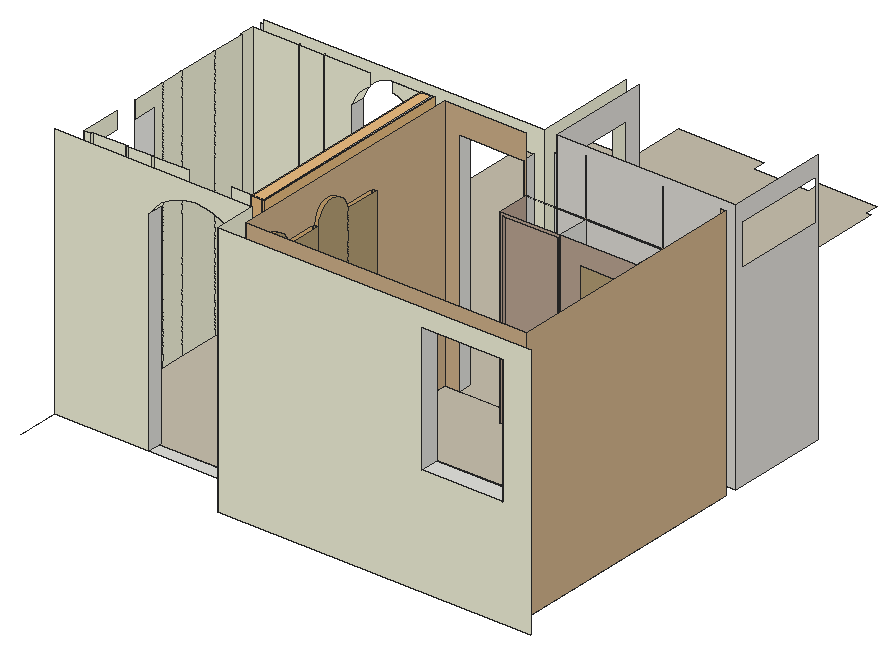
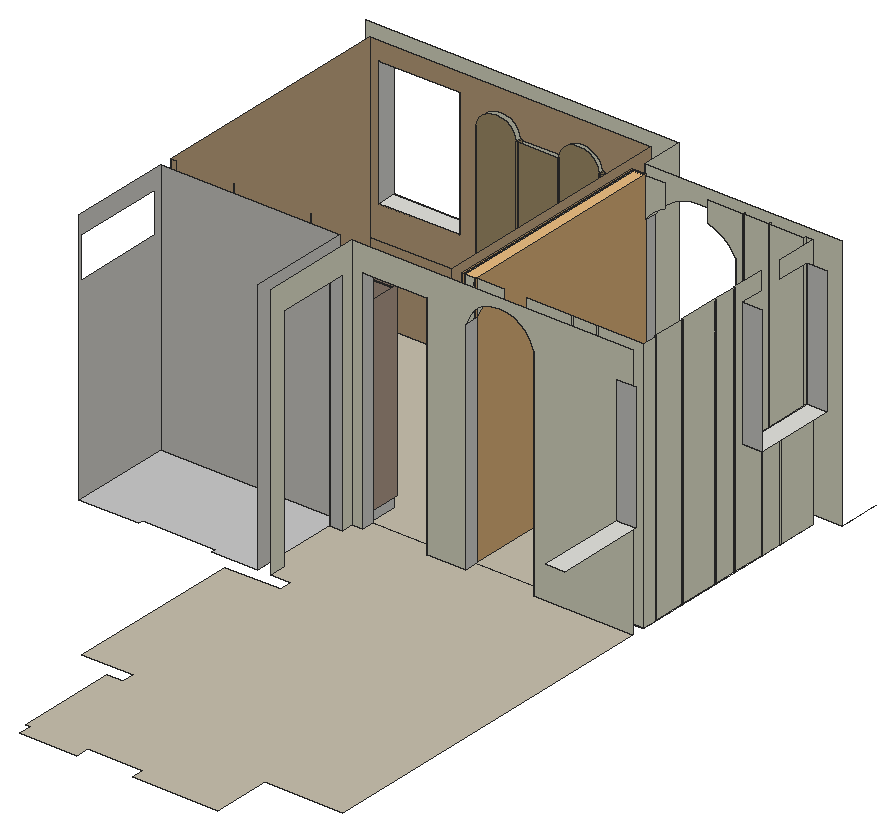
# SketchUp Ruby script. Lengths in inches.
U = 1.inch
M = Sketchup.active_model
def pt(a) = Geom::Point3d.new(a.map { |v| v * U })
def face(e, loops, mat)
  f = e.add_face(loops[0].map { |a| pt(a) })
  loops[1..].each { |l| e.add_face(l.map { |a| pt(a) }).erase! }
  f.material = f.back_material = mat if mat
  f
end
# faces: each face lists its corners as indices into pts; further lists are holes
def faces(e, pts, list, mat = nil) = list.each { |f| face(e, (f[0].is_a?(Array) ? f : [f]).map { |l| l.map { |i| pts[i] } }, mat) }
# xy, xz, yz: faces in a plane at the given z, y or x. An outline is a flat list of corners, or four numbers for a rectangle; further outlines are holes
def ring(l) = l.size == 4 ? [[l[0], l[1]], [l[2], l[1]], [l[2], l[3]], [l[0], l[3]]] : l.each_slice(2).to_a
def flat(e, list, mat, &to3) = list.each { |f| face(e, (f[0].is_a?(Array) ? f : [f]).map { |l| ring(l).map { |u, v| to3.(u, v) } }, mat) }
def xy(e, z, list, mat = nil) = flat(e, list, mat) { |x, y| [x, y, z] }
def xz(e, y, list, mat = nil) = flat(e, list, mat) { |x, z| [x, y, z] }
def yz(e, x, list, mat = nil) = flat(e, list, mat) { |y, z| [x, y, z] }
def lines(e, pts, list) = list.each { |a, b| e.add_line(pt(pts[a]), pt(pts[b])) }
# prism: a flat outline (further loops are holes) pulled along v
def prism(e, loops, v, mat = nil)
  f = face(e, loops, mat); d = Geom::Vector3d.new(v.map { |x| x * U })
  f.pushpull(f.normal.samedirection?(d) ? d.length : -d.length)
end
def box(e, o, s, mat = nil) = prism(e, [[o, [o[0] + s[0], o[1], o[2]], [o[0] + s[0], o[1] + s[1], o[2]], [o[0], o[1] + s[1], o[2]]]], [0, 0, s[2]], mat)
def at(x, y, z, deg = 0) = Geom::Transformation.translation(pt([x, y, z])) * Geom::Transformation.rotation(ORIGIN, Z_AXIS, deg.degrees)
def axes(o, x, y, z) = Geom::Transformation.new([*x, 0, *y, 0, *z, 0, *pt(o).to_a, 1])
def part(name) = M.definitions.add(name)
# library, detail: a bought-in or finely detailed component or shape, given as its bounding box
def library(name, o, s) = part(name).tap { |d| box(d.entities, o, s) }
def detail(e, o, s) = box(e.add_group.entities, o, s)
def put(e, d, t, mat = nil) = e.add_instance(d, t).tap { |i| i.material = mat if mat }
def group(e, t, mat = nil) = e.add_group.tap { |g| g.transformation = t; g.material = mat if mat }.entities
root = M.entities
M.materials.add("[0035_Tan]").color = [210, 180, 140]
M.materials.add("[0049_Beige]").color = [245, 245, 220]
M.materials.add("[0119_RosyBrown]").color = [188, 166, 148]
M.materials.add("[Marble Carrara Gold Floor Tile]").color = [225, 223, 217]
M.materials.add("[Ornate Tile 01]").color = [202, 202, 202]
M.materials.add("[Tile Canvas]1").color = [199, 192, 173]
M.materials.add("[Wallpaper Thin Brown Stripes]").color = [182, 160, 118]
c1 = library("Group\#5",[-5.3125,0,0],[6.3125,100,120])
xy(root,0,[[44.53,20,88.38,26]])
xy(root,0,[[88.38,26,93,26.8125]],"[0049_Beige]")
xy(root,0,[[147,132,231,132,231,180,203.125,180,203.125,177.6875,168.74,177.6875,168.74,180,147,180]],"[Ornate Tile 01]")
xy(root,0,[[99,9,231,9,231,126,228.5625,126,228.5625,112.75,137,112.75,137,126,136,126,136,132,141,132,141,137.75,147,137.75,147,172.25,141,172.25,141,180,131.5,180,131.5,186,157.6875,186,157.6875,270,133.48,270,133.48,276,141,276,141,324,138.73,324,138.73,330,112,330,112,324,86,324,86,330,45.9375,330,45.9375,302.26,9,302.26,9,132,55.625,132,55.625,125.5625,42.53,125.5625,42.53,126,42.33,126,42.33,125.5625,30.76,125.5625,30.76,126,30.5625,126,30.5625,125.5625,9,125.5625,9,118.43,9.5,118.43,9.5,102.75,9,102.75,9,102.55,9.5,102.55,9.5,83.3,9,83.3,9,83.1,9.5,83.1,9.5,71.98,9,71.98,9,71.78,9.5,71.78,9.5,56.09,9,56.09,9,55.9,9.25,55.9,9.25,45.39,9,45.39,9,45.1875,9.25,45.1875,9.25,26,12.5625,26,12.5625,26.8125,29.05,26.8125,29.05,26,29.25,26,29.25,26.8125,41.05,26.8125,41.05,26,41.25,26,41.25,26.8125,44.53,26.8125,44.53,26,88.38,26,88.38,26.8125,93,26.8125,93,126,88.16,126,88.16,125.5625,87.5,125.5625,87.5,132,105.75,132,105.75,126,99,126]],"[Tile Canvas]1")
xy(root,4.5,[[137,111,165.0625,112.75],[165.15,111,201.29,112.75],[201.375,111,228.5625,112.75],[165.0625,112.75,165.15,126],[201.29,112.75,201.375,126]])
xy(root,5.71,[[138.21,111,163.85,112.1875]],"[0119_RosyBrown]")
xy(root,5.75,[[202.62,111,227.31,112.1875]],"[0119_RosyBrown]")
xy(root,32.08,[[121.62,9,140.32,11.25],[160.12,9,178.82,11.75],[99,14,101.1875,31],[99,48.8,101.25,65.8]],"[Wallpaper Thin Brown Stripes]")
xy(root,51.4375,[[188.875,0,226.8125,9]])
xy(root,52.1875,[[0,29.375,9.25,29.375,9.25,45.1875,9,45.1875,9,45.39,9.25,45.39,9.25,55.9,9,55.9,9,56.09,9.5,56.09,9.5,67.375,0,67.375],[0,141.25,9,183]])
xz(root,0,[[[93,0,240,120],[188.875,51.4375,226.8125,111.6875]]],"[0049_Beige]")
xz(root,9,[[[99,0,231,120],[188.875,51.4375,226.8125,111.6875],[150.11,22.95,152.64,23.27,154.99,24.19,156.97,25.66,158.4375,27.56,159.29,29.76,159.46,32.08,159.46,102.01,140.76,102.01,140.76,32.08,140.93,29.76,141.78,27.56,143.25,25.66,145.23,24.19,147.58,23.27],[111.83,22.95,114.36,23.27,116.71,24.19,118.6875,25.66,120.16,27.56,121.01,29.76,121.18,32.08,121.18,102.01,102.48,102.01,102.48,32.08,102.65,29.76,103.5,27.56,104.97,25.66,106.95,24.19,109.3,23.27],[160.12,32.08,178.82,32.08,178.82,102.01,178.4,104.125,177.41,106.08,175.91,107.74,174.01,109.01,171.8125,109.8,169.47,110.08,167.125,109.8,164.93,109.01,163.03,107.74,161.53,106.08,160.54,104.125,160.12,102.01],[121.62,32.08,140.32,32.08,140.32,102.01,139.89,104.12,138.89,106.06,137.4,107.71,135.49,108.98,133.31,109.77,130.97,110.04,128.63,109.77,126.44,108.98,124.54,107.71,123.04,106.06,122.05,104.12,121.62,102.01]]],"[0035_Tan]")
xz(root,11.25,[[111.83,22.95,109.3,23.27,106.95,24.19,104.97,25.66,103.5,27.56,102.65,29.76,102.48,32.08,102.48,102.01,121.18,102.01,121.18,32.08,121.01,29.76,120.16,27.56,118.6875,25.66,116.71,24.19,114.36,23.27],[150.11,22.95,147.58,23.27,145.23,24.19,143.25,25.66,141.78,27.56,140.93,29.76,140.76,32.08,140.76,102.01,159.46,102.01,159.46,32.08,159.29,29.76,158.4375,27.56,156.97,25.66,154.99,24.19,152.64,23.27],[121.62,32.08,121.62,102.01,122.05,104.12,123.04,106.06,124.54,107.71,126.44,108.98,128.63,109.77,130.97,110.04,133.31,109.77,135.49,108.98,137.4,107.71,138.89,106.06,139.89,104.12,140.32,102.01,140.32,32.08]],"[Wallpaper Thin Brown Stripes]")
xz(root,11.75,[[160.12,32.08,160.12,102.01,160.54,104.125,161.53,106.08,163.03,107.74,164.93,109.01,167.125,109.8,169.47,110.08,171.8125,109.8,174.01,109.01,175.91,107.74,177.41,106.08,178.4,104.125,178.82,102.01,178.82,32.08]],"[Wallpaper Thin Brown Stripes]")
xz(root,14,[[99,32.08,101.1875,101.92]],"[Wallpaper Thin Brown Stripes]")
xz(root,20,[[0,0,44.53,0,44.53,100.0625,47.16,103.53,50.33,106.5,53.95,108.91,57.92,110.68,62.125,111.76,66.46,112.125,70.79,111.76,75,110.68,78.97,108.91,82.59,106.5,85.75,103.53,88.38,100.0625,88.38,0,93,0,93,120,0,120]],"[0049_Beige]")
xz(root,26,[[9.25,0,12.36,120],[12.36,0,12.5625,120],[29.05,0,29.25,120],[41.05,0,41.25,120]],"[0049_Beige]")
xz(root,26.8125,[[12.5625,0,29.05,120],[29.25,0,41.05,120],[41.25,0,41.25,120,57.6,120,57.6,110.54,53.95,108.91,50.33,106.5,47.16,103.53,44.53,100.0625,44.53,0],[88.38,0,88.38,100.0625,85.75,103.53,82.59,106.5,78.97,108.91,78.0625,109.3125,78.0625,120,93,120,93,0]],"[0049_Beige]")
xz(root,29.375,[[0,52.1875,9.25,111.75]])
xz(root,31,[[99,32.08,101.1875,101.92]],"[Wallpaper Thin Brown Stripes]")
xz(root,31.4,[[99,32.08,101.25,101.92]],"[Wallpaper Thin Brown Stripes]")
xz(root,45.1875,[[9,0,9.25,52.1875]],"[0049_Beige]")
xz(root,45.39,[[9,0,9.25,52.1875]],"[0049_Beige]")
xz(root,48.4,[[99,32.08,101.25,101.92]],"[Wallpaper Thin Brown Stripes]")
xz(root,48.8,[[99,32.08,101.25,101.92]],"[Wallpaper Thin Brown Stripes]")
xz(root,55.9,[[9,0,9.25,52.1875]],"[0049_Beige]")
xz(root,56.09,[[9,0,9.5,52.1875]],"[0049_Beige]")
xz(root,65.8,[[99,32.08,101.25,101.92]],"[Wallpaper Thin Brown Stripes]")
xz(root,66.3,[[99,32.08,101.25,101.92]],"[Wallpaper Thin Brown Stripes]")
xz(root,67.375,[[0,52.1875,9.5,111.75]])
xz(root,71.78,[[9,0,9.5,120]],"[0049_Beige]")
xz(root,71.98,[[9,0,9.5,120]],"[0049_Beige]")
xz(root,83.1,[[9,0,9.5,120]],"[0049_Beige]")
xz(root,83.1,[[99,32.08,101.25,101.92]],"[Wallpaper Thin Brown Stripes]")
xz(root,83.3,[[9,0,9.5,120]],"[0049_Beige]")
xz(root,102.55,[[9,0,9.5,120]],"[0049_Beige]")
xz(root,102.75,[[9,0,9.5,120]],"[0049_Beige]")
xz(root,111,[[[137,4.5,165.0625,93.41],[138.21,5.71,163.85,92.2]],[[165.15,4.5,201.29,93.41],[174.41,13.76,192.03,84.15]],[[201.375,4.5,228.5625,93.41],[202.62,5.75,227.31,92.17]]],"[0119_RosyBrown]")
xz(root,111,[[174.41,13.76,192.03,84.15]],"[Wallpaper Thin Brown Stripes]")
xz(root,112.1875,[[138.21,5.71,163.85,92.2],[202.62,5.75,227.31,92.17]],"[0119_RosyBrown]")
xz(root,112.75,[[137,0,228.5625,4.5]])
xz(root,118.43,[[9,0,9.5,120]],"[0049_Beige]")
xz(root,125.5625,[[9,0,30.5625,120],[30.76,0,42.33,120],[42.53,0,55.625,0,55.625,103.25,56.89,106.64,58.86,109.68,61.45,112.21,64.21,113.91,64.01,113.91,64.01,120,42.53,120],[87.5,0,88.16,0,88.16,120,74.6,120,74.6,115.35,75.16,115.29,78.59,114.11,81.67,112.21,84.26,109.68,86.24,106.64,87.5,103.25]],"[0049_Beige]")
xz(root,126,[[99,0,105.75,0,105.75,108,136,108,136,0,137,0,137,93.41,165.0625,93.41,165.0625,4.5,165.15,4.5,165.15,93.41,201.29,93.41,201.29,4.5,201.375,4.5,201.375,93.41,228.5625,93.41,228.5625,0,231,0,231,120,228.5625,120,228.5625,93.5625,201.375,93.5625,201.375,119,201.6875,119,201.6875,120,201.29,120,201.29,93.5625,165.15,93.5625,165.15,119,165.46,119,165.46,120,165.0625,120,165.0625,93.5625,137,93.5625,137,120,99,120]],"[0035_Tan]")
xz(root,126,[[30.5625,0,30.76,120],[42.33,0,42.53,120],[88.16,0,88.36,120],[88.36,0,93,120]],"[0049_Beige]")
xz(root,132,[[9,0,9,120,141,120,141,0,136,0,136,108,105.75,108,105.75,0,87.5,0,87.5,103.25,86.24,106.64,84.26,109.68,81.67,112.21,78.59,114.11,75.16,115.29,71.5625,115.6875,67.96,115.29,64.54,114.11,61.45,112.21,58.86,109.68,56.89,106.64,55.625,103.25,55.625,0]],"[0049_Beige]")
xz(root,132,[[147,0,231,120]],"[Marble Carrara Gold Floor Tile]")
xz(root,137.75,[[141,0,147,108]])
xz(root,141.25,[[0,52.1875,9,111.75]])
yz(root,9,[[45.1875,0,45.39,52.1875],[55.9,0,56.09,52.1875],[71.78,0,71.98,120],[83.1,0,83.3,120],[102.55,0,102.75,120],
  [118.43,0,118.62,120],[118.62,0,125.5625,120]],"[0049_Beige]")
yz(root,9.25,[[26,0,45.1875,0,45.1875,52.1875,29.375,52.1875,29.375,111.75,45.1875,111.75,45.1875,120,26,120],[45.39,0,55.9,52.1875]],"[0049_Beige]")
yz(root,9.5,[[56.09,0,71.78,0,71.78,120,56.09,120,56.09,111.75,67.375,111.75,67.375,52.1875,56.09,52.1875],[71.98,0,83.1,120],[83.3,0,102.55,120],[102.75,0,118.43,120]],"[0049_Beige]")
yz(root,12.5625,[[26,0,26.8125,120]],"[0049_Beige]")
yz(root,29.05,[[26,0,26.8125,120]],"[0049_Beige]")
yz(root,29.25,[[26,0,26.8125,120]],"[0049_Beige]")
yz(root,30.5625,[[125.5625,0,126,120]],"[0049_Beige]")
yz(root,30.76,[[125.5625,0,126,120]],"[0049_Beige]")
yz(root,41.05,[[26,0,26.8125,120]],"[0049_Beige]")
yz(root,41.25,[[26,0,26.8125,120]],"[0049_Beige]")
yz(root,42.33,[[125.5625,0,126,120]],"[0049_Beige]")
yz(root,42.53,[[125.5625,0,126,120]],"[0049_Beige]")
yz(root,44.53,[[20,0,26.8125,100.0625]])
yz(root,55.625,[[125.5625,0,132,103.25]])
yz(root,87.5,[[125.5625,0,132,103.25]])
yz(root,88.16,[[125.5625,0,126,120]],"[0049_Beige]")
yz(root,88.38,[[20,0,26,100.0625]])
yz(root,88.38,[[26,0,26.8125,100.0625]],"[0049_Beige]")
yz(root,93,[[26.8125,0,126,120]])
yz(root,93,[[0,0,20,120],[26,0,26.8125,120]],"[0049_Beige]")
yz(root,99,[[[9,0,126,120],[39.9,22.91,37.59,23.23,35.45,24.16,33.65,25.64,32.3125,27.55,31.54,29.75,31.4,32.08,31.4,101.92,48.4,101.92,48.4,32.08,48.26,29.75,47.49,27.55,46.15,25.64,44.35,24.16,42.21,23.23],[74.7,22.91,72.4,23.23,70.27,24.16,68.48,25.64,67.16,27.56,66.42,29.76,66.3,32.08,66.3,101.92,83.1,101.92,83.1,32.08,82.98,29.76,82.23,27.56,80.92,25.64,79.125,24.16,77,23.23],[14,32.08,14,101.92,14.37,104.05,15.27,106.01,16.625,107.6875,18.36,108.97,20.36,109.77,22.5,110.04,24.64,109.77,26.64,108.97,28.375,107.6875,29.73,106.01,30.63,104.05,31,101.92,31,32.08],[48.8,32.08,48.8,101.92,49.17,104.05,50.07,106.01,51.42,107.6875,53.16,108.97,55.16,109.77,57.3,110.04,59.4375,109.77,61.44,108.97,63.18,107.6875,64.53,106.01,65.43,104.05,65.8,101.92,65.8,32.08]]],"[0035_Tan]")
yz(root,101.1875,[[14,32.08,31,32.08,31,101.92,30.63,104.05,29.73,106.01,28.375,107.6875,26.64,108.97,24.64,109.77,22.5,110.04,20.36,109.77,18.36,108.97,16.625,107.6875,15.27,106.01,14.37,104.05,14,101.92]],"[Wallpaper Thin Brown Stripes]")
yz(root,101.25,[[39.9,22.91,42.21,23.23,44.35,24.16,46.15,25.64,47.49,27.55,48.26,29.75,48.4,32.08,48.4,101.92,31.4,101.92,31.4,32.08,31.54,29.75,32.3125,27.55,33.65,25.64,35.45,24.16,37.59,23.23],[74.7,22.91,77,23.23,79.125,24.16,80.92,25.64,82.23,27.56,82.98,29.76,83.1,32.08,83.1,101.92,66.3,101.92,66.3,32.08,66.42,29.76,67.16,27.56,68.48,25.64,70.27,24.16,72.4,23.23],[48.8,32.08,65.8,32.08,65.8,101.92,65.43,104.05,64.53,106.01,63.18,107.6875,61.44,108.97,59.4375,109.77,57.3,110.04,55.16,109.77,53.16,108.97,51.42,107.6875,50.07,106.01,49.17,104.05,48.8,101.92]],"[Wallpaper Thin Brown Stripes]")
yz(root,102.48,[[9,32.08,11.25,102.01]],"[Wallpaper Thin Brown Stripes]")
yz(root,105.75,[[126,0,132,108]])
yz(root,121.18,[[9,32.08,11.25,102.01]],"[Wallpaper Thin Brown Stripes]")
yz(root,121.62,[[9,32.08,11.25,102.01]],"[Wallpaper Thin Brown Stripes]")
yz(root,136,[[126,0,132,108]])
yz(root,137,[[112.75,0,126,4.5]])
yz(root,137,[[111,4.5,126,93.41]],"[0119_RosyBrown]")
yz(root,138.21,[[111,5.71,112.1875,92.2]],"[0119_RosyBrown]")
yz(root,140.32,[[9,32.08,11.25,102.01]],"[Wallpaper Thin Brown Stripes]")
yz(root,140.76,[[9,32.08,11.25,102.01]],"[Wallpaper Thin Brown Stripes]")
yz(root,141,[[132,0,132,120,180,120,180,0,172.25,0,172.25,108,137.75,108,137.75,0]],"[0049_Beige]")
yz(root,147,[[132,0,137.75,0,137.75,108,172.25,108,172.25,0,180,0,180,120,132,120]],"[Marble Carrara Gold Floor Tile]")
yz(root,159.46,[[9,32.08,11.25,102.01]],"[Wallpaper Thin Brown Stripes]")
yz(root,160.12,[[9,32.08,11.75,102.01]],"[Wallpaper Thin Brown Stripes]")
yz(root,163.85,[[111,5.71,112.1875,92.2]],"[0119_RosyBrown]")
yz(root,165.0625,[[111,4.5,126,93.41]])
yz(root,165.15,[[111,4.5,126,93.41]])
yz(root,178.82,[[9,32.08,11.75,102.01]],"[Wallpaper Thin Brown Stripes]")
yz(root,188.875,[[0,51.4375,9,111.6875]])
yz(root,201.29,[[111,4.5,126,93.41]])
yz(root,201.375,[[111,4.5,126,93.41]])
yz(root,202.62,[[111,5.75,112.1875,92.17]],"[0119_RosyBrown]")
yz(root,226.8125,[[0,51.4375,9,111.6875]])
yz(root,227.31,[[111,5.75,112.1875,92.17]],"[0119_RosyBrown]")
yz(root,228.5625,[[112.75,0,126,4.5],[111,4.5,126,93.41]])
yz(root,231,[[9,0,126,120]],"[0035_Tan]")
yz(root,231,[[[132,0,180,120],[135.375,92,178.8125,111.25]]],"[Marble Carrara Gold Floor Tile]")
p = [[99,37.59,23.23],[99,39.9,22.91],[101.25,39.9,22.91],[101.25,37.59,23.23],[99,42.21,23.23],[101.25,42.21,23.23],
  [99,72.4,23.23],[99,74.7,22.91],[101.25,74.7,22.91],[101.25,72.4,23.23],[99,77,23.23],[101.25,77,23.23],
  [111.83,9,22.95],[109.3,9,23.27],[109.3,11.25,23.27],[111.83,11.25,22.95],[114.36,9,23.27],[114.36,11.25,23.27],
  [150.11,9,22.95],[147.58,9,23.27],[147.58,11.25,23.27],[150.11,11.25,22.95],[152.64,9,23.27],[152.64,11.25,23.27],
  [99,35.45,24.16],[101.25,35.45,24.16],[99,44.35,24.16],[101.25,44.35,24.16],[99,70.27,24.16],[101.25,70.27,24.16],
  [99,79.125,24.16],[101.25,79.125,24.16],[106.95,9,24.19],[106.95,11.25,24.19],[116.71,9,24.19],[116.71,11.25,24.19],
  [145.23,9,24.19],[145.23,11.25,24.19],[154.99,9,24.19],[154.99,11.25,24.19],[104.97,9,25.66],[104.97,11.25,25.66],
  [118.6875,9,25.66],[118.6875,11.25,25.66],[143.25,9,25.66],[143.25,11.25,25.66],[156.97,9,25.66],[156.97,11.25,25.66],
  [99,33.65,25.64],[101.25,33.65,25.64],[99,46.15,25.64],[101.25,46.15,25.64],[99,68.48,25.64],[101.25,68.48,25.64],
  [99,80.92,25.64],[101.25,80.92,25.64],[99,32.3125,27.55],[101.25,32.3125,27.55],[99,47.49,27.55],[101.25,47.49,27.55],
  [99,67.16,27.56],[101.25,67.16,27.56],[99,82.23,27.56],[101.25,82.23,27.56],[103.5,9,27.56],[103.5,11.25,27.56],
  [120.16,9,27.56],[120.16,11.25,27.56],[141.78,9,27.56],[141.78,11.25,27.56],[158.4375,9,27.56],[158.4375,11.25,27.56],
  [99,31.54,29.75],[101.25,31.54,29.75],[99,48.26,29.75],[101.25,48.26,29.75],[102.65,9,29.76],[102.65,11.25,29.76],
  [121.01,9,29.76],[121.01,11.25,29.76],[140.93,9,29.76],[140.93,11.25,29.76],[159.29,9,29.76],[159.29,11.25,29.76],
  [99,66.42,29.76],[101.25,66.42,29.76],[99,82.98,29.76],[101.25,82.98,29.76],[99,31.4,32.08],[101.25,31.4,32.08],
  [99,48.4,32.08],[101.25,48.4,32.08],[102.48,9,32.08],[102.48,11.25,32.08],[121.18,9,32.08],[121.18,11.25,32.08],
  [140.76,9,32.08],[140.76,11.25,32.08],[159.46,9,32.08],[159.46,11.25,32.08],[99,66.3,32.08],[101.25,66.3,32.08],
  [99,83.1,32.08],[101.25,83.1,32.08],[0,20,0],[0,0,0],[136,126,0],[134.99,126,0]]
faces(root,p,[[0,1,2,3],[1,4,5,2],[6,7,8,9],[7,10,11,8],[12,13,14,15],[16,12,15,17],[18,19,20,21],[22,18,21,23],
  [24,0,3,25],[4,26,27,5],[28,6,9,29],[10,30,31,11],[13,32,33,14],[34,16,17,35],[19,36,37,20],[38,22,23,39],
  [32,40,41,33],[42,34,35,43],[36,44,45,37],[46,38,39,47],[48,24,25,49],[26,50,51,27],[52,28,29,53],[30,54,55,31],
  [56,48,49,57],[50,58,59,51],[60,52,53,61],[54,62,63,55],[40,64,65,41],[66,42,43,67],[44,68,69,45],[70,46,47,71],
  [72,56,57,73],[58,74,75,59],[64,76,77,65],[78,66,67,79],[68,80,81,69],[82,70,71,83],[84,60,61,85],[62,86,87,63],
  [88,72,73,89],[74,90,91,75],[76,92,93,77],[94,78,79,95],[80,96,97,81],[98,82,83,99],[100,84,85,101],[86,102,103,87]],"[Wallpaper Thin Brown Stripes]")
lines(root,p,[[104,105],[106,107]])
g1 = group(root,at(99,9,0))
p = [[132,117,0],[132,0,0],[0,0,0],[0,117,0],[6.75,117,0],[40.1875,117,0]]
lines(g1,p,[[0,1],[1,2],[2,3],[3,4],[4,5],[5,0]])
g2 = group(root,at(9,26,0))
p = [[78.5,100,0],[84,100,0],[46.625,100,0],[0,100,0],[0,0,0],[35.53,0,0],
  [79.38,0,0],[84,0,0]]
lines(g2,p,[[0,1],[2,0],[3,2],[4,3],[5,4],[6,5],[7,6],[1,7]])
put(root,c1,at(93,26,0))
